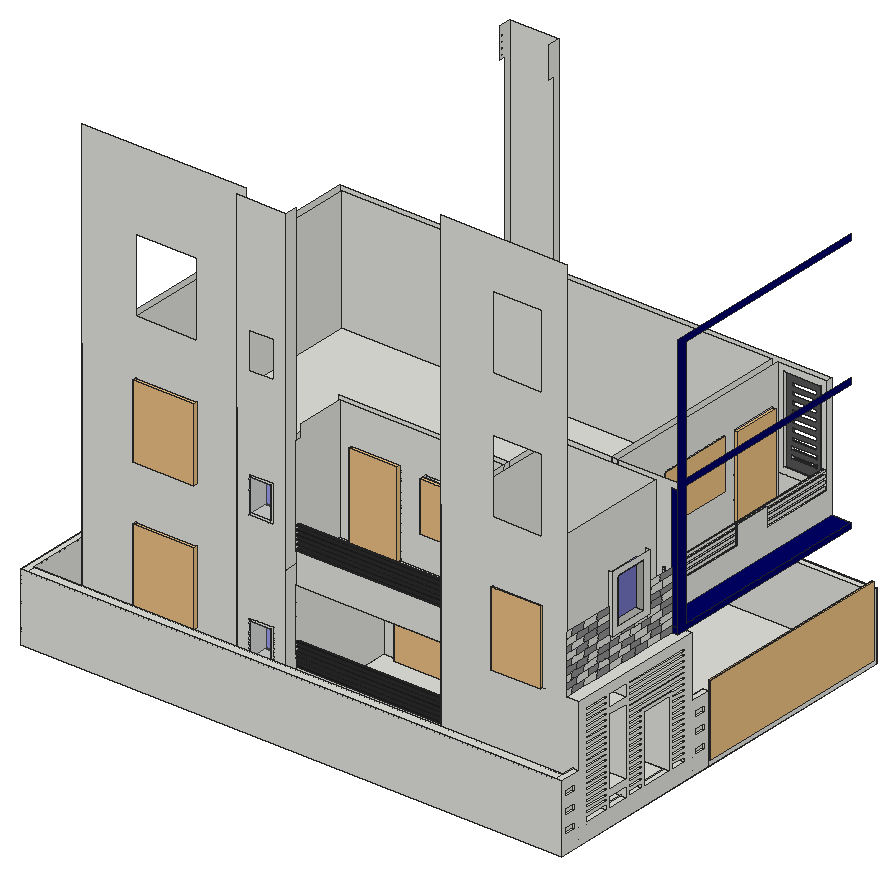
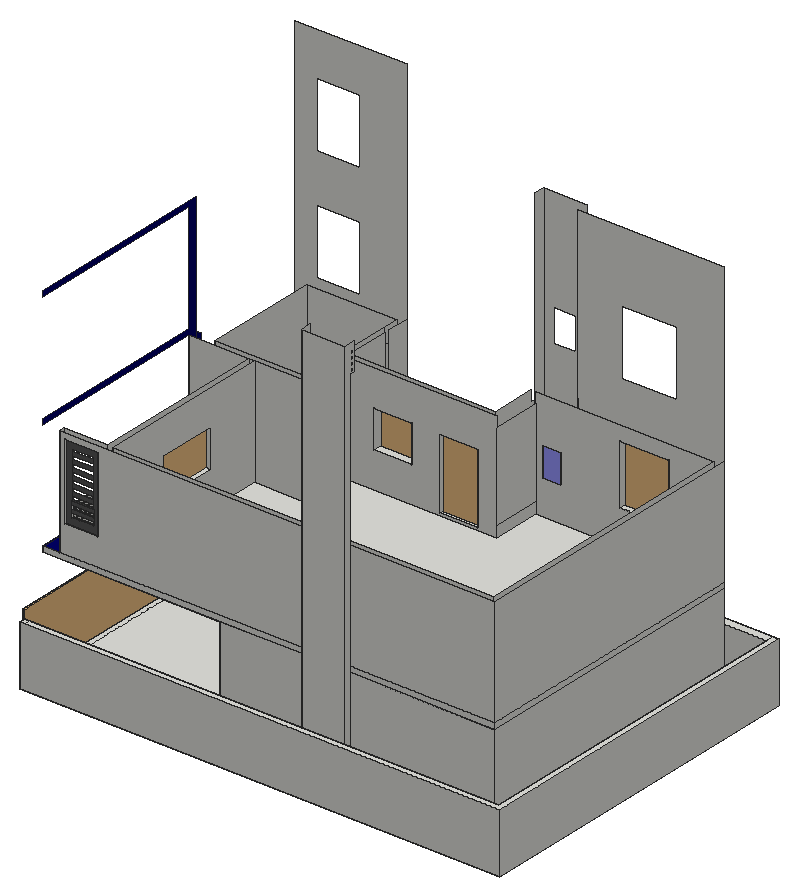
# SketchUp Ruby script. Lengths in inches.
U = 1.inch
M = Sketchup.active_model
def pt(a) = Geom::Point3d.new(a.map { |v| v * U })
def face(e, loops, mat)
  f = e.add_face(loops[0].map { |a| pt(a) })
  loops[1..].each { |l| e.add_face(l.map { |a| pt(a) }).erase! }
  f.material = f.back_material = mat if mat
  f
end
# faces: each face lists its corners as indices into pts; further lists are holes
def faces(e, pts, list, mat = nil) = list.each { |f| face(e, (f[0].is_a?(Array) ? f : [f]).map { |l| l.map { |i| pts[i] } }, mat) }
# xy, xz, yz: faces in a plane at the given z, y or x. An outline is a flat list of corners, or four numbers for a rectangle; further outlines are holes
def ring(l) = l.size == 4 ? [[l[0], l[1]], [l[2], l[1]], [l[2], l[3]], [l[0], l[3]]] : l.each_slice(2).to_a
def flat(e, list, mat, &to3) = list.each { |f| face(e, (f[0].is_a?(Array) ? f : [f]).map { |l| ring(l).map { |u, v| to3.(u, v) } }, mat) }
def xy(e, z, list, mat = nil) = flat(e, list, mat) { |x, y| [x, y, z] }
def xz(e, y, list, mat = nil) = flat(e, list, mat) { |x, z| [x, y, z] }
def yz(e, x, list, mat = nil) = flat(e, list, mat) { |y, z| [x, y, z] }
def lines(e, pts, list) = list.each { |a, b| e.add_line(pt(pts[a]), pt(pts[b])) }
# prism: a flat outline (further loops are holes) pulled along v
def prism(e, loops, v, mat = nil)
  f = face(e, loops, mat); d = Geom::Vector3d.new(v.map { |x| x * U })
  f.pushpull(f.normal.samedirection?(d) ? d.length : -d.length)
end
def box(e, o, s, mat = nil) = prism(e, [[o, [o[0] + s[0], o[1], o[2]], [o[0] + s[0], o[1] + s[1], o[2]], [o[0], o[1] + s[1], o[2]]]], [0, 0, s[2]], mat)
def at(x, y, z, deg = 0) = Geom::Transformation.translation(pt([x, y, z])) * Geom::Transformation.rotation(ORIGIN, Z_AXIS, deg.degrees)
def axes(o, x, y, z) = Geom::Transformation.new([*x, 0, *y, 0, *z, 0, *pt(o).to_a, 1])
def part(name) = M.definitions.add(name)
# library, detail: a bought-in or finely detailed component or shape, given as its bounding box
def library(name, o, s) = part(name).tap { |d| box(d.entities, o, s) }
def detail(e, o, s) = box(e.add_group.entities, o, s)
def put(e, d, t, mat = nil) = e.add_instance(d, t).tap { |i| i.material = mat if mat }
def group(e, t, mat = nil) = e.add_group.tap { |g| g.transformation = t; g.material = mat if mat }.entities
root = M.entities
M.materials.add("Glass_Basic_01").color = [0, 0, 0]
M.materials["Glass_Basic_01"].alpha = 0.25
M.materials.add("Glass_Basic_1").color = [161, 173, 186]
M.materials["Glass_Basic_1"].alpha = 0.25
M.materials.add("I02_Moonlit_Azure").color = [153, 153, 255]
M.materials.add("I08_Inkstorm").color = [0, 0, 102]
M.materials.add("M04_Stone_Frost").color = [142, 142, 142]
M.materials.add("M06_Steel_Smoke").color = [86, 86, 86]
M.materials.add("M08_Obsidian_Black").color = [30, 30, 30]
c1 = library("porta+4",[0.2,-5.42,1.33],[46.55,4.72,83.21])
c2 = library("Modern+Gate+1",[0,0,0],[118.11,1.97,78.74])
c3 = library("mesh-166",[-1553.69,-2604.3125,-42.18],[1702.88,1401.6,88.28])
c4 = part("Group17")
put(c4.entities,c3,at(294.66,859.51,3.5))
c5 = library("mesh-160",[-91.39,-1008.79,-36.9],[2366.42,1739.16,65.81])
c6 = part("Group4")
g1 = group(c6.entities,at(-5.75,-6.15,0))
put(g1,c5,axes([0,0,0],[1,0,0],[0,0,1],[0,-1,0]))
c7 = part("Balcony railing")
xy(c7.entities,0.4,[[0,0.79,160.5,2.29]])
xy(c7.entities,2.4,[[0,0.79,160.5,2.29]])
xy(c7.entities,4.59,[[0,0.79,160.5,2.29]])
xy(c7.entities,6.59,[[0,0.79,160.5,2.29]])
xy(c7.entities,8.79,[[0,0.79,160.5,2.29]])
xy(c7.entities,10.79,[[0,0.79,160.5,2.29]])
xy(c7.entities,12.98,[[0,0.79,160.5,2.29]])
xy(c7.entities,14.98,[[0,0.79,160.5,2.29]])
xy(c7.entities,17.17,[[0,0.79,160.5,2.29]])
xy(c7.entities,19.17,[[0,0.79,160.5,2.29]])
xy(c7.entities,21.36,[[0,0.79,160.5,2.29]])
xy(c7.entities,23.36,[[0,0.79,160.5,2.29]])
xz(c7.entities,0.79,[[0,0.4,160.5,2.4],[0,4.59,160.5,6.59],[0,8.79,160.5,10.79],[0,12.98,160.5,14.98],[0,17.17,160.5,19.17],
  [0,21.36,160.5,23.36]])
xz(c7.entities,2.29,[[0,0.4,160.5,2.4],[0,4.59,160.5,6.59],[0,8.79,160.5,10.79],[0,12.98,160.5,14.98],[0,17.17,160.5,19.17],
  [0,21.36,160.5,23.36]])
yz(c7.entities,0,[[[0,0,3,24],[0.79,21.36,2.29,23.36],[0.79,17.17,2.29,19.17],[0.79,12.98,2.29,14.98],[0.79,8.79,2.29,10.79],[0.79,4.59,2.29,6.59],[0.79,0.4,2.29,2.4]]])
yz(c7.entities,160.5,[[0.79,0.4,2.29,2.4],[0.79,4.59,2.29,6.59],[0.79,8.79,2.29,10.79],[0.79,12.98,2.29,14.98],[0.79,17.17,2.29,19.17],
  [0.79,21.36,2.29,23.36]])
c8 = library("mesh-162",[-1607.75,-1245.64,-53.98],[1739.16,1702.88,120.91])
c9 = part("Group9")
put(c9.entities,c8,at(0,0,0))
c10 = part("RAIL")
xy(c10.entities,0,[[0,0,2,195]])
xy(c10.entities,2.57,[[0,0,2,195]])
xy(c10.entities,5.14,[[0,0,2,195]])
xy(c10.entities,7.71,[[0,0,2,195]])
xy(c10.entities,10.29,[[0,0,2,195]])
xy(c10.entities,12.86,[[0,0,2,195]])
xy(c10.entities,15.43,[[0,0,2,195]])
xy(c10.entities,18,[[0,0,2,195]])
xz(c10.entities,0,[[0,2.57,2,5.14],[0,7.71,2,10.29],[0,12.86,2,15.43]])
xz(c10.entities,195,[[0,0,2,2.57],[0,5.14,2,7.71],[0,10.29,2,12.86],[0,15.43,2,18]])
yz(c10.entities,0,[[0,0,195,2.57],[0,5.14,195,7.71],[0,10.29,195,12.86],[0,15.43,195,18]])
yz(c10.entities,2,[[0,0,195,2.57],[0,5.14,195,7.71],[0,10.29,195,12.86],[0,15.43,195,18]])
xy(root,-6,[[0,0,528,384]])
xy(root,0,[[6,9,495,9,495,21,393,21,393,45,232.5,45,232.5,33,184.5,33,184.5,45,24,45,24,360,184.5,360,184.5,366,232.5,366,232.5,360,327,360,327,159,522,159,522,378,6,378],[495,9,522,21],[[393,21,393,45,232.5,45,232.5,33,184.5,33,184.5,45,33,45,33,51,226.5,51,226.5,153,33,153,33,45,24,45,24,360,184.5,360,184.5,366,232.5,366,232.5,360,327,360,327,159,522,159,522,150,495,150,495,153,399,153,399,27,495,27,495,30,522,30,522,21],[33,159,177,351],[183,159,321,351],[232.5,51,393,153]],[399,27,495,27,495,30,522,30,522,150,495,150,495,153,399,153],[33,51,226.5,153],
  [232.5,51,393,153],[33,159,177,351],[183,159,321,351],[522,180,528,378]])
xy(root,3,[[247.5,153,286.03,159],[286.03,153,289.5,159],[321,303,327,345]])
xy(root,10.67,[[522,30,528,55.44],[495,55.44,522,58.09],[522,55.44,528,58.09],[522,58.09,528,79.45],[495,79.45,522,82.5],
  [522,79.45,528,82.5],[522,82.5,528,98.4],[495,98.4,522,101.04],[522,98.4,528,101.04],[522,101.04,528,132.44],
  [495,132.44,522,134.68],[522,132.44,528,134.68],[522,134.68,528,150]])
xy(root,11.17,[[525,4.62,528,16.62],[525,162.94,528,174.94]])
xy(root,15.68,[[495,30,528,55.44],[495,82.5,528,98.4],[495,134.68,528,150]])
xy(root,17.17,[[525,4.62,528,16.62],[525,162.94,528,174.94]])
xy(root,18.19,[[495,30,528,55.44],[495,82.5,528,98.4],[495,134.68,528,150]])
xy(root,20.7,[[495,30,528,55.44],[495,82.5,528,98.4],[495,134.68,528,150]])
xy(root,21,[[495,58.09,528,79.45]])
xy(root,23.21,[[495,30,528,55.44],[495,82.5,528,98.4],[495,134.68,528,150]])
xy(root,25.72,[[495,30,528,55.44],[495,82.5,528,98.4],[495,134.68,528,150]])
xy(root,27,[[495,58.09,528,79.45]])
xy(root,27.84,[[525,4.62,528,16.62],[525,162.94,528,174.94]])
xy(root,28.22,[[495,30,528,55.44],[495,82.5,528,98.4],[495,134.68,528,150]])
xy(root,30.73,[[495,30,528,55.44],[495,82.5,528,98.4],[495,134.68,528,150]])
xy(root,33.24,[[495,30,528,55.44],[495,82.5,528,98.4],[495,134.68,528,150]])
xy(root,33.84,[[525,4.62,528,16.62],[525,162.94,528,174.94]])
xy(root,35.75,[[495,30,528,55.44],[495,82.5,528,98.4],[495,134.68,528,150]])
xy(root,36,[[232.5,45,393,51],[316.5,149,364.5,153]])
xy(root,38,[[198.5,33,218.5,51]])
xy(root,38.26,[[495,30,528,55.44],[495,82.5,528,98.4],[495,134.68,528,150]])
xy(root,39,[[79.5,45,133.5,51],[319.5,149,361.5,153],[321,219,327,285]])
xy(root,40.77,[[495,30,528,55.44],[495,82.5,528,98.4],[495,134.68,528,150]])
xy(root,43.27,[[495,30,528,55.44],[495,82.5,528,98.4],[495,134.68,528,150]])
xy(root,43.95,[[525,4.62,528,16.62],[525,162.94,528,174.94]])
xy(root,45.78,[[495,30,528,55.44],[495,82.5,528,98.4],[495,134.68,528,150]])
xy(root,48.29,[[495,30,528,55.44],[495,82.5,528,98.4],[495,134.68,528,150]])
xy(root,49.95,[[525,4.62,528,16.62],[525,162.94,528,174.94]])
xy(root,50.8,[[495,30,528,55.44],[495,82.5,528,98.4],[495,134.68,528,150]])
xy(root,53.31,[[495,30,528,55.44],[495,82.5,528,98.4],[495,134.68,528,150]])
xy(root,55.82,[[495,30,528,55.44],[495,82.5,528,98.4],[495,134.68,528,150]])
xy(root,58.32,[[495,30,528,55.44],[495,82.5,528,98.4],[495,134.68,528,150]])
xy(root,60,[[0,0,6,0,6,378,522,378,522,384,0,384],[6,0,522,9],[522,0,528,21],[522,159,528,180],[522,378,528,384]])
xy(root,60.83,[[495,30,528,55.44],[495,82.5,528,98.4],[495,134.68,528,150]])
xy(root,63.34,[[495,30,528,55.44],[495,82.5,528,98.4],[495,134.68,528,150]])
xy(root,65.85,[[495,30,528,55.44],[495,82.5,528,98.4],[495,134.68,528,150]])
xy(root,68.36,[[495,30,528,55.44],[495,82.5,528,98.4],[495,134.68,528,150]])
xy(root,70,[[198.5,33,218.5,51]])
xy(root,70.87,[[495,30,528,55.44],[495,82.5,528,98.4],[495,134.68,528,150]])
xy(root,73.375,[[495,30,528,55.44],[495,82.5,528,98.4],[495,134.68,528,150]])
xy(root,75.88,[[495,30,528,55.44],[495,82.5,528,98.4],[495,134.68,528,150]])
xy(root,76.35,[[495,101.04,528,132.44]])
xy(root,78.39,[[495,30,528,55.44],[495,82.5,528,98.4],[495,134.68,528,150]])
xy(root,79.35,[[495,98.4,528,134.68]])
xy(root,80.9,[[495,30,528,55.44],[495,82.5,528,150]])
xy(root,81,[[319.5,149,361.5,153],[247.5,153,289.5,159],[321,219,327,285],[321,303,327,345]])
xy(root,83.41,[[495,30,528,55.44],[495,82.5,528,150]])
xy(root,84,[[316.5,149,364.5,153]])
xy(root,85.92,[[495,30,528,55.44],[495,82.5,528,150]])
xy(root,88.42,[[495,30,528,55.44],[495,82.5,528,150]])
xy(root,90.93,[[495,30,528,55.44],[495,82.5,528,150]])
xy(root,93,[[495,58.09,528,79.45]])
xy(root,93.44,[[495,30,528,55.44],[495,82.5,528,150]])
xy(root,95.95,[[495,30,528,55.44],[495,82.5,528,150]])
xy(root,98.46,[[495,30,528,55.44],[495,82.5,528,150]])
xy(root,99,[[495,58.09,528,79.45]])
xy(root,100.97,[[495,30,528,55.44],[495,82.5,528,150]])
xy(root,103.47,[[495,30,528,55.44],[495,82.5,528,150]])
xy(root,105,[[79.5,45,133.5,51]])
xy(root,105.98,[[495,30,528,55.44],[495,82.5,528,150]])
xy(root,108,[[232.5,45,393,51]])
xy(root,108.49,[[495,30,528,55.44],[495,82.5,528,150]])
xy(root,111,[[495,30,528,33.9],[495,33.9,528,42.77],[495,42.77,528,46.8],[495,46.8,528,55.44],[495,58.09,528,59.7],
  [495,59.7,495,67.45,528,66.15,528,59.7],[528,66.15,495,67.45,495,72.6,528,72.6],[495,72.6,528,73.41],[495,73.41,528,79.45],[495,82.5,528,88.72],
  [495,88.72,528,98.4],[495,98.4,528,104.04],[495,104.04,528,111.3],[495,111.3,528,119.36],[495,119.36,528,124.2],
  [495,124.2,528,129.44],[495,129.44,528,134.68],[495,134.68,528,137.1],[495,137.1,528,150]])
xy(root,120,[[516,21,528,21,528,159,522,159,522,150,516,150],[399,27,495,51],[24,51,33,153],[33,51,226.5,153],[232.5,51,393,153],
  [393,51,399,153],[399,51,495,153],[24,159,33,351],[33,159,177,351],[183,159,321,351],
  [327,159,522,360],[24,351,177,360]])
xy(root,123,[[447,21,489,27],[399,27,498,153]])
xy(root,126,[[30,51,226.5,51,226.5,105,393,105,393,159,450,159,450,354,30,354],[232.5,51,393,99],[456,159,498,354]])
xy(root,126,[[504,159,522,360]],"I08_Inkstorm")
xy(root,128,[[247.5,99,289.5,105]])
xy(root,129,[[450,303,456,345]])
xy(root,138,[[232.5,45,393,51]])
xy(root,150,[[498,159,499,354],[499,159,500,354],[500,159,502,354],[502,159,503,354],[503,159,504,244.5],
  [503,280.5,504,354]])
xy(root,151.5,[[516,72.6,520,117.43]])
xy(root,156,[[462,354,498,356],[462,356,498,358],[462,358,498,360]])
xy(root,157.86,[[512,78.73,520,110.73]])
xy(root,162,[[316.5,95,364.5,99]])
xy(root,164,[[198.5,33,218.5,51],[468,356,492,358]])
xy(root,165,[[79.5,45,133.5,51],[319.5,95,361.5,105],[450,219,456,285]])
xy(root,168,[[503,244.5,504,256.5],[503,256.5,504,280.5],[468,356,492,358]])
xy(root,172,[[468,356,492,358]])
xy(root,176,[[468,356,492,358]])
xz(root,0,[[0,-6,528,60]])
xz(root,4.62,[[525,11.17,528,17.17],[525,27.84,528,33.84],[525,43.95,528,49.95]])
xz(root,9,[[6,0,495,60],[495,0,522,60]])
xz(root,16.62,[[525,11.17,528,17.17],[525,27.84,528,33.84],[525,43.95,528,49.95]])
xz(root,21,[[[393,0,522,0,522,60,528,60,528,120,516,120,516,498,393,498],[444,252,492,324],[444,378,492,450],[444,120,492,192]],[[444,120,492,192],[447,123,489,189]]])
xz(root,27,[[399,0,495,120],[399,123,399,246,498,246,498,123,489,123,489,189,447,189,447,123]])
xz(root,30,[[495,0,522,10.67],[495,10.67,528,13.17],[495,13.17,528,15.68],[495,18.19,528,20.7],[495,23.21,528,25.72],
  [495,28.22,528,30.73],[495,33.24,528,35.75],[495,38.26,528,40.77],[495,43.27,528,45.78],[495,48.29,528,50.8],
  [495,53.31,528,55.82],[495,58.32,528,60.83],[495,63.34,528,65.85],[495,68.36,528,70.87],[495,73.375,528,75.88],
  [495,78.39,528,80.9],[495,83.41,528,85.92],[495,88.42,528,90.93],[495,93.44,528,95.95],[495,98.46,528,100.97],
  [495,103.47,528,105.98],[495,108.49,528,111]])
xz(root,33,[[[184.5,0,232.5,438],[196.5,36,220.5,72],[196.5,162,220.5,198],[196.5,288,220.5,324]],[[196.5,36,220.5,72],[198.5,38,218.5,70]],[[196.5,162,220.5,198],[198.5,164,218.5,196]]])
xz(root,33,[[198.5,38,218.5,70],[198.5,164,218.5,196]],"Glass_Basic_1")
xz(root,45,[[[24,0,184.5,438],[76.5,36,136.5,108],[76.5,162,136.5,234],[76.5,288,136.5,360]],[232.5,0,393,36],[[76.5,36,136.5,108],[79.5,39,133.5,105]],[232.5,108,393,138],[[76.5,162,136.5,234],[79.5,165,133.5,231]]])
xz(root,51,[[[33,0,226.5,120],[79.5,39,133.5,105],[198.5,38,218.5,70]],[232.5,0,393,36],[232.5,108,393,120],[[30,126,226.5,246],[79.5,165,133.5,231],[198.5,164,218.5,196]],[232.5,126,393,138]])
xz(root,51,[[198.5,38,218.5,70],[198.5,164,218.5,196]],"I02_Moonlit_Azure")
xz(root,55.44,[[495,10.67,528,15.68],[495,15.68,528,18.19],[495,18.19,528,20.7],[495,20.7,528,23.21],[495,23.21,528,25.72],
  [495,25.72,528,28.22],[495,28.22,528,30.73],[495,30.73,528,33.24],[495,33.24,528,35.75],[495,35.75,528,38.26],
  [495,38.26,528,40.77],[495,40.77,528,43.27],[495,43.27,528,45.78],[495,45.78,528,48.29],[495,48.29,528,50.8],
  [495,50.8,528,53.31],[495,53.31,528,55.82],[495,55.82,528,58.32],[495,58.32,528,60.83],[495,60.83,528,63.34],
  [495,63.34,528,65.85],[495,65.85,528,68.36],[495,68.36,528,70.87],[495,70.87,528,73.375],[495,73.375,528,75.88],
  [495,75.88,528,78.39],[495,78.39,528,80.9],[495,80.9,528,83.41],[495,83.41,528,85.92],[495,85.92,528,88.42],
  [495,88.42,528,90.93],[495,90.93,528,93.44],[495,93.44,528,95.95],[495,95.95,528,98.46],[495,98.46,528,100.97],
  [495,100.97,528,103.47],[495,103.47,528,105.98],[495,105.98,528,108.49],[495,108.49,528,111]])
xz(root,58.09,[[495,10.67,528,21],[495,27,528,93],[495,99,528,111]])
xz(root,72.6,[[516,151.5,520,208.2]])
xz(root,78.73,[[512,157.86,520,201.86]])
xz(root,79.45,[[495,10.67,528,21],[495,27,528,93],[495,99,528,111]])
xz(root,82.5,[[495,10.67,528,13.17],[495,13.17,528,15.68],[495,18.19,528,20.7],[495,23.21,528,25.72],[495,28.22,528,30.73],
  [495,33.24,528,35.75],[495,38.26,528,40.77],[495,43.27,528,45.78],[495,48.29,528,50.8],[495,53.31,528,55.82],
  [495,58.32,528,60.83],[495,63.34,528,65.85],[495,68.36,528,70.87],[495,73.375,528,75.88],[495,78.39,528,80.9],
  [495,83.41,528,85.92],[495,88.42,528,90.93],[495,93.44,528,95.95],[495,98.46,528,100.97],[495,103.47,528,105.98],
  [495,108.49,528,111]])
xz(root,95,[[[316.5,162,364.5,210],[319.5,165,361.5,207]]])
xz(root,98.4,[[495,10.67,528,15.68],[495,15.68,528,18.19],[495,18.19,528,20.7],[495,20.7,528,23.21],[495,23.21,528,25.72],
  [495,25.72,528,28.22],[495,28.22,528,30.73],[495,30.73,528,33.24],[495,33.24,528,35.75],[495,35.75,528,38.26],
  [495,38.26,528,40.77],[495,40.77,528,43.27],[495,43.27,528,45.78],[495,45.78,528,48.29],[495,48.29,528,50.8],
  [495,50.8,528,53.31],[495,53.31,528,55.82],[495,55.82,528,58.32],[495,58.32,528,60.83],[495,60.83,528,63.34],
  [495,63.34,528,65.85],[495,65.85,528,68.36],[495,68.36,528,70.87],[495,70.87,528,73.375],[495,73.375,528,75.88],
  [495,75.88,528,78.39],[495,78.39,528,79.35]])
xz(root,99,[[244.5,125,292.5,126],[[232.5,126,244.5,126,244.5,209,292.5,209,292.5,126,393,126,393,246,232.5,246],[316.5,162,364.5,210]],[[244.5,126,292.5,209],[247.5,128,289.5,206]]])
xz(root,101.04,[[495,10.67,528,76.35]])
xz(root,105,[[[226.5,126,393,246],[247.5,128,289.5,206],[319.5,165,361.5,207]]])
xz(root,110.73,[[512,157.86,520,201.86]])
xz(root,117.43,[[516,151.5,520,208.2]])
xz(root,132.44,[[495,10.67,528,76.35]])
xz(root,134.68,[[495,10.67,528,15.68],[495,15.68,528,18.19],[495,18.19,528,20.7],[495,20.7,528,23.21],[495,23.21,528,25.72],
  [495,25.72,528,28.22],[495,28.22,528,30.73],[495,30.73,528,33.24],[495,33.24,528,35.75],[495,35.75,528,38.26],
  [495,38.26,528,40.77],[495,40.77,528,43.27],[495,43.27,528,45.78],[495,45.78,528,48.29],[495,48.29,528,50.8],
  [495,50.8,528,53.31],[495,53.31,528,55.82],[495,55.82,528,58.32],[495,58.32,528,60.83],[495,60.83,528,63.34],
  [495,63.34,528,65.85],[495,65.85,528,68.36],[495,68.36,528,70.87],[495,70.87,528,73.375],[495,73.375,528,75.88],
  [495,75.88,528,78.39],[495,78.39,528,79.35]])
xz(root,149,[[[316.5,36,364.5,84],[319.5,39,361.5,81]]])
xz(root,150,[[495,0,522,10.67],[495,10.67,528,13.17],[495,13.17,528,15.68],[495,18.19,528,20.7],[495,23.21,528,25.72],
  [495,28.22,528,30.73],[495,33.24,528,35.75],[495,38.26,528,40.77],[495,43.27,528,45.78],[495,48.29,528,50.8],
  [495,53.31,528,55.82],[495,58.32,528,60.83],[495,63.34,528,65.85],[495,68.36,528,70.87],[495,73.375,528,75.88],
  [495,78.39,528,80.9],[495,80.9,528,83.41],[495,83.41,528,85.92],[495,85.92,528,88.42],[495,88.42,528,90.93],
  [495,90.93,528,93.44],[495,93.44,528,95.95],[495,95.95,528,98.46],[495,98.46,528,100.97],[495,100.97,528,103.47],
  [495,103.47,528,105.98],[495,105.98,528,108.49],[495,108.49,528,111]])
xz(root,150,[[516,120,522,126],[516,126,522,246]],"I08_Inkstorm")
xz(root,153,[[238.03,-1,286.03,0],[33,0,226.5,120],[226.5,0,232.5,120],[[232.5,0,244.5,0,244.5,84,292.5,84,292.5,0,393,0,393,120,232.5,120],[316.5,36,364.5,84]],[[244.5,0,292.5,84],[247.5,3,289.5,81]],
  [399,0,495,120],[319.5,39,361.5,81],[399,123,498,246]])
xz(root,159,[[33,0,177,120],[[183,0,321,120],[247.5,3,289.5,81]],[327,0,327,120,528,120,528,60,522,60,522,0],[393,126,450,246],[450,126,456,246],
  [456,126,456,246,522,246,522,126,504,126,504,150,502,150,502,168,500,168,500,150,498,150,498,126]])
xz(root,162.94,[[525,11.17,528,17.17],[525,27.84,528,33.84],[525,43.95,528,49.95]])
xz(root,174.94,[[525,11.17,528,17.17],[525,27.84,528,33.84],[525,43.95,528,49.95]])
xz(root,180,[[522,0,528,60]])
xz(root,219,[[321,39,327,81],[450,165,456,207]])
xz(root,244.5,[[503,150,504,168]])
xz(root,280.5,[[503,150,504,168]])
xz(root,285,[[321,39,327,81],[450,165,456,207]])
xz(root,303,[[321,3,327,81],[450,129,456,207]])
xz(root,345,[[321,3,327,81],[450,129,456,207]])
xz(root,351,[[33,0,177,120],[183,0,321,120]])
xz(root,354,[[30,126,450,246],[456,126,498,150],[[456,150,504,246],[462,156,498,240]]])
xz(root,356,[[[462,156,498,240],[468,228,492,232],[468,220,492,224],[468,212,492,216],[468,204,492,208],[468,196,492,200],[468,188,492,192],[468,180,492,184],[468,172,492,176],[468,164,492,168]]],"M06_Steel_Smoke")
xz(root,358,[[[462,156,498,240],[468,164,492,232]],[468,168,492,172],[468,176,492,180]],"M06_Steel_Smoke")
xz(root,360,[[24,0,184.5,120],[232.5,0,327,120],[24,120,184.5,126],[232.5,120,522,126],[24,126,184.5,246],
  [[232.5,126,504,246],[462,156,498,240]]])
xz(root,366,[[184.5,0,232.5,444]])
xz(root,378,[[6,0,522,60],[522,0,528,60]])
xz(root,384,[[0,-6,528,60]])
yz(root,0,[[0,-6,384,60]])
yz(root,6,[[9,0,378,60]])
yz(root,24,[[45,0,360,120],[45,120,360,126],[45,126,360,246]])
yz(root,30,[[51,126,354,246]])
yz(root,33,[[51,0,153,120],[159,0,351,120]])
yz(root,79.5,[[45,39,51,105],[45,165,51,231]])
yz(root,133.5,[[45,39,51,105],[45,165,51,231]])
yz(root,177,[[159,0,351,120]])
yz(root,183,[[159,0,351,120]])
yz(root,184.5,[[33,0,45,126],[[360,0,360,414,354,414,354,444,366,444,366,0],[356,433.14,358,436],[356,427.43,358,430.29],[356,421.71,358,424.57],[356,416,358,418.86]],[33,126,45,252]])
yz(root,198.5,[[33,38,51,70],[33,164,51,196]])
yz(root,218.5,[[33,38,51,70],[33,164,51,196]])
yz(root,226.5,[[51,0,153,12],[51,12,153,108],[51,108,153,120],[51,126,105,138],[51,138,105,234]])
yz(root,232.5,[[33,0,45,126],[51,0,153,0,153,120,51,120,51,108,45,108,45,48,48,48,48,36,51,36],[360,0,366,7.45],[[360,7.45,366,7.45,366,444,354,444,354,414,360,414],[356,433.14,358,436],[356,427.43,358,430.29],[356,421.71,358,424.57],[356,416,358,418.86]],[33,126,45,438],
  [51,126,99,126,99,246,51,246,51,234,45,234,45,138,51,138]])
yz(root,247.5,[[153,3,159,81],[99,128,105,206]])
yz(root,289.5,[[153,3,159,81],[99,128,105,206]])
yz(root,316.5,[[149,36,153,84],[95,162,99,210]])
yz(root,319.5,[[149,39,153,81],[95,165,105,207]])
yz(root,321,[[[159,0,351,120],[303,3,345,81],[219,39,285,81]]])
yz(root,327,[[[159,0,300,0,300,84,348,84,348,0,360,0,360,120,159,120],[216,36,288,84]],[[300,0,348,84],[303,3,345,81]],[[216,36,288,84],[219,39,285,81]]])
yz(root,361.5,[[149,39,153,81],[95,165,105,207]])
yz(root,364.5,[[149,36,153,84],[95,162,99,210]])
yz(root,393,[[21,0,45,246],[51,0,153,120],[45,36,51,108],[45,126,51,138],[51,126,99,246],
  [99,126,105,246],[105,126,159,246],[45,138,51,234]])
yz(root,399,[[27,0,153,120],[27,123,45,246],[45,123,153,246]])
yz(root,447,[[21,123,27,189]])
yz(root,450,[[[159,126,354,246],[303,129,345,207],[219,165,285,207]]])
yz(root,456,[[[159,126,300,126,300,210,348,210,348,126,354,126,354,246,159,246],[216,162,288,210]],[[300,126,348,210],[303,129,345,207]],[[216,162,288,210],[219,165,285,207]]])
yz(root,462,[[354,156,356,240],[358,156,360,240]])
yz(root,468,[[356,164,358,168],[356,172,358,176]])
yz(root,489,[[21,123,27,189]])
yz(root,492,[[356,164,358,168],[356,172,358,176]])
yz(root,495,[[[27,0,27,120,153,120,153,0,150,0,150,15.68,134.68,15.68,134.68,18.19,150,18.19,150,20.7,134.68,20.7,134.68,23.21,150,23.21,150,25.72,134.68,25.72,134.68,28.22,150,28.22,150,30.73,134.68,30.73,134.68,33.24,150,33.24,150,35.75,134.68,35.75,134.68,38.26,150,38.26,150,40.77,134.68,40.77,134.68,43.27,150,43.27,150,45.78,134.68,45.78,134.68,48.29,150,48.29,150,50.8,134.68,50.8,134.68,53.31,150,53.31,150,55.82,134.68,55.82,134.68,58.32,150,58.32,150,60.83,134.68,60.83,134.68,63.34,150,63.34,150,65.85,134.68,65.85,134.68,68.36,150,68.36,150,70.87,134.68,70.87,134.68,73.375,150,73.375,150,75.88,134.68,75.88,134.68,78.39,150,78.39,150,80.9,82.5,80.9,82.5,78.39,98.4,78.39,98.4,75.88,82.5,75.88,82.5,73.375,98.4,73.375,98.4,70.87,82.5,70.87,82.5,68.36,98.4,68.36,98.4,65.85,82.5,65.85,82.5,63.34,98.4,63.34,98.4,60.83,82.5,60.83,82.5,58.32,98.4,58.32,98.4,55.82,82.5,55.82,82.5,53.31,98.4,53.31,98.4,50.8,82.5,50.8,82.5,48.29,98.4,48.29,98.4,45.78,82.5,45.78,82.5,43.27,98.4,43.27,98.4,40.77,82.5,40.77,82.5,38.26,98.4,38.26,98.4,35.75,82.5,35.75,82.5,33.24,98.4,33.24,98.4,30.73,82.5,30.73,82.5,28.22,98.4,28.22,98.4,25.72,82.5,25.72,82.5,23.21,98.4,23.21,98.4,20.7,82.5,20.7,82.5,18.19,98.4,18.19,98.4,15.68,82.5,15.68,82.5,10.67,79.45,10.67,79.45,21,58.09,21,58.09,27,79.45,27,79.45,93,58.09,93,58.09,99,79.45,99,79.45,111,58.09,111,58.09,10.67,55.44,10.67,55.44,15.68,30,15.68,30,0],[82.5,103.47,150,105.98],[82.5,108.49,150,111],[82.5,93.44,150,95.95],[82.5,88.42,150,90.93],[82.5,83.41,150,85.92],[82.5,98.46,150,100.97],[30,103.47,55.44,105.98],[30,93.44,55.44,95.95],[30,88.42,55.44,90.93],[30,108.49,55.44,111],[30,83.41,55.44,85.92],[30,78.39,55.44,80.9],[30,73.375,55.44,75.88],[30,68.36,55.44,70.87],[30,18.19,55.44,20.7],[30,63.34,55.44,65.85],[30,58.32,55.44,60.83],[30,53.31,55.44,55.82],[30,48.29,55.44,50.8],[30,43.27,55.44,45.78],[30,38.26,55.44,40.77],[30,33.24,55.44,35.75],[30,28.22,55.44,30.73],[30,23.21,55.44,25.72],[30,98.46,55.44,100.97]],[98.4,10.67,98.4,79.35,129.44,79.35,129.44,76.35,101.04,76.35,101.04,10.67],[132.44,10.67,132.44,76.35,129.44,76.35,129.44,79.35,134.68,79.35,134.68,10.67]])
yz(root,498,[[27,123,153,246],[159,126,354,150],[354,156,356,240],[358,156,360,240]])
yz(root,503,[[244.5,150,256.5,168],[256.5,150,280.5,168]])
yz(root,504,[[159,126,360,126,360,246,354,246,354,150,280.5,150,280.5,168,244.5,168,244.5,150,159,150]])
yz(root,512,[[78.73,157.86,110.73,201.86]],"I02_Moonlit_Azure")
yz(root,516,[[21,120,27.45,126.3],[42.77,120,58.09,126.3],[73.41,120,88.72,126.3],[119.36,120,134.68,126.3],[33.9,126.3,46.8,132.6],
  [59.7,126.3,72.6,132.6],[85.5,126.3,98.4,132.6],[111.3,126.3,124.2,132.6],[137.1,126.3,150,132.6],[21,132.6,27.45,138.9],
  [42.77,132.6,58.09,138.9],[73.41,132.6,88.72,138.9],[104.04,132.6,119.36,138.9],[134.68,132.6,150,138.9],[46.8,138.9,59.7,145.2],
  [85.5,138.9,98.4,145.2],[98.4,138.9,111.3,145.2],[124.2,138.9,137.1,145.2],[27.45,145.2,42.77,151.5],[58.09,145.2,73.41,151.5],
  [73.41,145.2,88.72,151.5],[104.04,145.2,119.36,151.5],[119.36,145.2,134.68,151.5],[21,151.5,33.9,157.8],[46.8,151.5,59.7,157.8],
  [117.43,151.5,124.2,157.8],[137.1,151.5,150,157.8],[27.45,157.8,42.77,164.1],[72.6,157.8,73.41,164.1],[117.43,157.8,119.36,164.1],
  [21,164.1,33.9,170.4],[59.7,164.1,72.6,170.4],[124.2,164.1,137.1,170.4],[137.1,164.1,150,170.4],[21,170.4,27.45,176.7],
  [42.77,170.4,58.09,176.7],[72.6,170.4,73.41,176.7],[117.43,170.4,119.36,176.7],[119.36,170.4,134.68,176.7]])
yz(root,516,[[27.45,120,42.77,126.3],[58.09,120,73.41,126.3],[88.72,120,104.04,126.3],[104.04,120,119.36,126.3],[134.68,120,150,126.3],
  [21,126.3,33.9,132.6],[46.8,126.3,59.7,132.6],[72.6,126.3,85.5,132.6],[98.4,126.3,111.3,132.6],[124.2,126.3,137.1,132.6],
  [27.45,132.6,42.77,138.9],[58.09,132.6,73.41,138.9],[88.72,132.6,104.04,138.9],[119.36,132.6,134.68,138.9],[21,138.9,33.9,145.2],
  [33.9,138.9,46.8,145.2],[59.7,138.9,72.6,145.2],[72.6,138.9,85.5,145.2],[111.3,138.9,124.2,145.2],[137.1,138.9,150,145.2],
  [21,145.2,27.45,151.5],[42.77,145.2,58.09,151.5],[88.72,145.2,104.04,151.5],[134.68,145.2,150,151.5],[33.9,151.5,46.8,157.8],
  [59.7,151.5,72.6,157.8],[124.2,151.5,137.1,157.8],[21,157.8,27.45,164.1],[42.77,157.8,58.09,164.1],[58.09,157.8,72.6,164.1],
  [119.36,157.8,134.68,164.1],[134.68,157.8,150,164.1],[33.9,164.1,46.8,170.4],[46.8,164.1,59.7,170.4],[117.43,164.1,124.2,170.4],
  [27.45,170.4,42.77,176.7],[58.09,170.4,72.6,176.7],[134.68,170.4,150,176.7]],"M04_Stone_Frost")
yz(root,520,[[[72.6,151.5,117.43,208.2],[78.73,157.86,110.73,201.86]]])
yz(root,520,[[78.73,157.86,110.73,201.86]],"Glass_Basic_01")
yz(root,522,[[9,0,21,60],[21,0,30,10.67],[30,0,150,9],[150,0,159,10.67],[159,0,180,60],
  [30,9,150,10.67]])
yz(root,522,[[150,120,360,120,360,126,159,126,159,246,360,246,360,252,159,252,159,372,360,372,360,378,150,378]],"I08_Inkstorm")
yz(root,525,[[4.62,11.17,16.62,17.17],[162.94,11.17,174.94,17.17],[4.62,27.84,16.62,33.84],[162.94,27.84,174.94,33.84],[4.62,43.95,16.62,49.95],
  [162.94,43.95,174.94,49.95]])
yz(root,528,[[[0,-6,180,-6,180,60,159,60,159,120,21,120,21,60,0,60],[101.04,10.67,132.44,76.35],[58.09,27,79.45,93],[58.09,99,79.45,111],[58.09,10.67,79.45,21],[82.5,103.47,150,105.98],[82.5,108.49,150,111],[82.5,93.44,150,95.95],[82.5,83.41,150,85.92],[82.5,88.42,150,90.93],[82.5,98.46,150,100.97],[82.5,78.39,82.5,80.9,150,80.9,150,78.39,134.68,78.39,134.68,79.35,98.4,79.35,98.4,78.39],[30,10.67,55.44,15.68],[82.5,10.67,98.4,15.68],[134.68,10.67,150,15.68],[4.62,43.95,16.62,49.95],[162.94,43.95,174.94,49.95],[162.94,27.84,174.94,33.84],[4.62,27.84,16.62,33.84],[162.94,11.17,174.94,17.17],[4.62,11.17,16.62,17.17],[30,88.42,55.44,90.93],[30,93.44,55.44,95.95],[30,103.47,55.44,105.98],[30,108.49,55.44,111],[30,83.41,55.44,85.92],[30,73.375,55.44,75.88],[30,78.39,55.44,80.9],[30,18.19,55.44,20.7],[30,68.36,55.44,70.87],[30,23.21,55.44,25.72],[30,28.22,55.44,30.73],[30,33.24,55.44,35.75],[30,38.26,55.44,40.77],[30,43.27,55.44,45.78],[30,48.29,55.44,50.8],[30,53.31,55.44,55.82],[30,58.32,55.44,60.83],[30,63.34,55.44,65.85],[30,98.46,55.44,100.97],[82.5,38.26,98.4,40.77],[82.5,43.27,98.4,45.78],[82.5,48.29,98.4,50.8],[82.5,53.31,98.4,55.82],[82.5,58.32,98.4,60.83],[82.5,63.34,98.4,65.85],[82.5,68.36,98.4,70.87],[82.5,73.375,98.4,75.88],[82.5,33.24,98.4,35.75],[82.5,18.19,98.4,20.7],[82.5,23.21,98.4,25.72],[82.5,28.22,98.4,30.73],[134.68,63.34,150,65.85],[134.68,68.36,150,70.87],[134.68,73.375,150,75.88],[134.68,58.32,150,60.83],[134.68,18.19,150,20.7],[134.68,23.21,150,25.72],[134.68,28.22,150,30.73],[134.68,33.24,150,35.75],[134.68,38.26,150,40.77],[134.68,43.27,150,45.78],[134.68,48.29,150,50.8],[134.68,53.31,150,55.82]],[180,-6,384,-6,384,60,378,60,378,0,180,0]])
p = [[33,159,0],[33,153,0],[183,351,0],[177,351,0],[183,351,120],[183,360,120],
  [321,351,120],[321,360,120],[495,51,120],[504,51,120],[495,153,120],[504,153,120],
  [495,27,120],[495,21,120],[522,21,10.67],[528,21,10.67],[522,21,0],[528,21,0],
  [522,159,0],[528,159,0],[522,159,10.67],[528,159,10.67],[522,30,9],[528,30,9],
  [492,21,120]]
lines(root,p,[[0,1],[2,3],[4,5],[6,7],[8,9],[10,11],[12,13],[14,15],[16,17],[18,19],[20,21],[22,23],
  [13,24]])
put(root,c1,at(325.16,299.8,-1.37,90))
put(root,c1,at(244.3,154.84,-1.37))
put(root,c2,axes([529.97,180,0],[0,1.6764,0],[-1,0,0],[0,0,0.88]))
put(root,c4,axes([328.91,147.61,95.8],[-0.02795,0,0],[0,0,0.03438],[0,0.02795,0]))
put(root,c6,axes([327.7,220.43,63.84],[0,0.02969,0],[-0.02283,0,0],[0,0,0.0276]))
put(root,c7,at(232.5,45,36),"M08_Obsidian_Black")
put(root,c4,axes([92.05,43.05,125.57],[-0.03504,0,0],[0,0,0.05118],[0,0.03937,0]))
put(root,c9,axes([456.89,20.72,186.51],[0,0,0.04175],[-0.02819,0,0],[0,-0.02087,0]))
put(root,c1,at(454.16,299.8,124.63,90))
put(root,c1,at(244.3,100.84,125.17))
put(root,c7,at(232.5,45,138),"M08_Obsidian_Black")
put(root,c10,at(500,159,150))
put(root,c4,axes([328.91,93.05,221.81],[-0.02795,0,0],[0,0,0.03441],[0,0.03937,0]))
put(root,c6,axes([456.7,218.95,189.87],[0,0.03037,0],[-0.02283,0,0],[0,0,0.02763]))
put(root,c4,axes([92.05,43.05,251.57],[-0.03504,0,0],[0,0,0.05118],[0,0.03937,0]))
